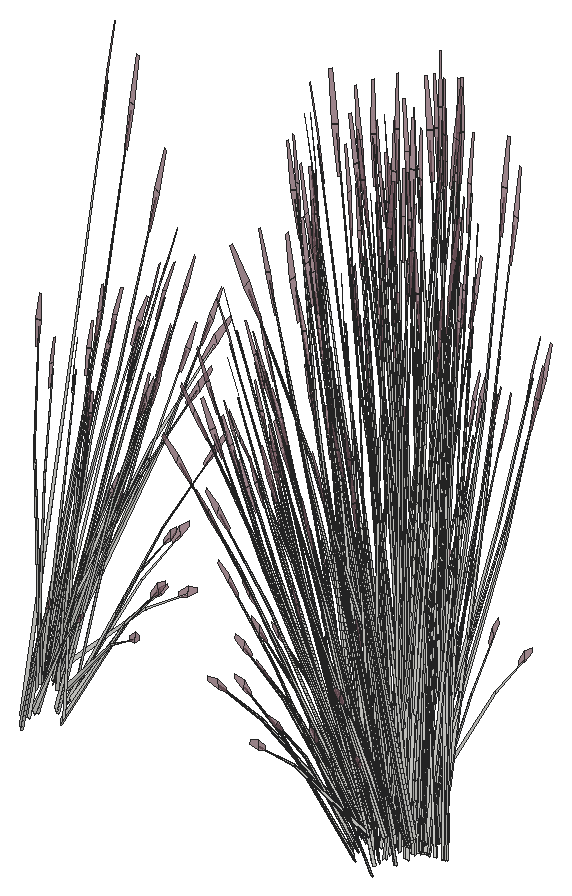
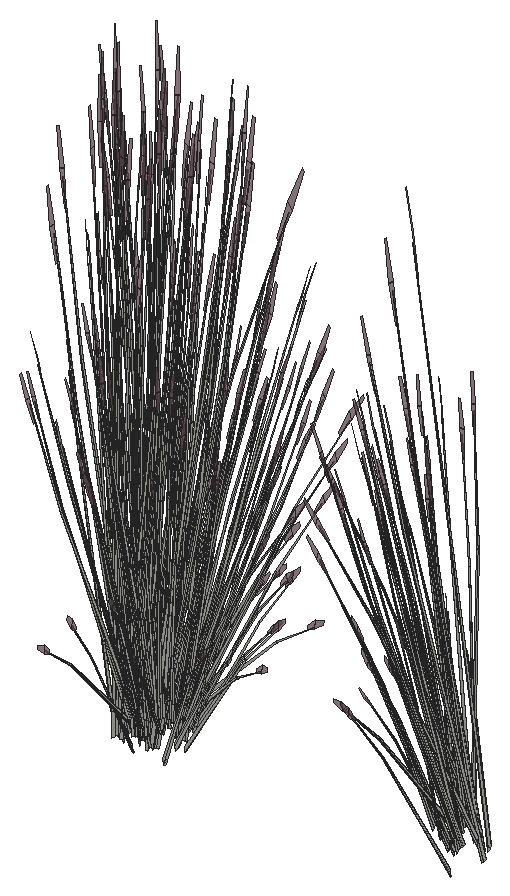
# SketchUp Ruby script. Lengths in inches.
U = 1.inch
M = Sketchup.active_model
def pt(a) = Geom::Point3d.new(a.map { |v| v * U })
def face(e, loops, mat)
  f = e.add_face(loops[0].map { |a| pt(a) })
  loops[1..].each { |l| e.add_face(l.map { |a| pt(a) }).erase! }
  f.material = f.back_material = mat if mat
  f
end
# faces: each face lists its corners as indices into pts; further lists are holes
def faces(e, pts, list, mat = nil) = list.each { |f| face(e, (f[0].is_a?(Array) ? f : [f]).map { |l| l.map { |i| pts[i] } }, mat) }
# xy, xz, yz: faces in a plane at the given z, y or x. An outline is a flat list of corners, or four numbers for a rectangle; further outlines are holes
def ring(l) = l.size == 4 ? [[l[0], l[1]], [l[2], l[1]], [l[2], l[3]], [l[0], l[3]]] : l.each_slice(2).to_a
def flat(e, list, mat, &to3) = list.each { |f| face(e, (f[0].is_a?(Array) ? f : [f]).map { |l| ring(l).map { |u, v| to3.(u, v) } }, mat) }
def xy(e, z, list, mat = nil) = flat(e, list, mat) { |x, y| [x, y, z] }
def xz(e, y, list, mat = nil) = flat(e, list, mat) { |x, z| [x, y, z] }
def yz(e, x, list, mat = nil) = flat(e, list, mat) { |y, z| [x, y, z] }
def lines(e, pts, list) = list.each { |a, b| e.add_line(pt(pts[a]), pt(pts[b])) }
# prism: a flat outline (further loops are holes) pulled along v
def prism(e, loops, v, mat = nil)
  f = face(e, loops, mat); d = Geom::Vector3d.new(v.map { |x| x * U })
  f.pushpull(f.normal.samedirection?(d) ? d.length : -d.length)
end
def box(e, o, s, mat = nil) = prism(e, [[o, [o[0] + s[0], o[1], o[2]], [o[0] + s[0], o[1] + s[1], o[2]], [o[0], o[1] + s[1], o[2]]]], [0, 0, s[2]], mat)
def at(x, y, z, deg = 0) = Geom::Transformation.translation(pt([x, y, z])) * Geom::Transformation.rotation(ORIGIN, Z_AXIS, deg.degrees)
def axes(o, x, y, z) = Geom::Transformation.new([*x, 0, *y, 0, *z, 0, *pt(o).to_a, 1])
def part(name) = M.definitions.add(name)
# library, detail: a bought-in or finely detailed component or shape, given as its bounding box
def library(name, o, s) = part(name).tap { |d| box(d.entities, o, s) }
def detail(e, o, s) = box(e.add_group.entities, o, s)
def put(e, d, t, mat = nil) = e.add_instance(d, t).tap { |i| i.material = mat if mat }
def group(e, t, mat = nil) = e.add_group.tap { |g| g.transformation = t; g.material = mat if mat }.entities
root = M.entities
M.materials.add("LightPink_Translucent").color = [144, 107, 117]
M.materials["LightPink_Translucent"].alpha = 0.75
c1 = part("blade")
p = [[2.15,0.21,22],[0,0.17,0],[0.09,0.45,0],[2.18,0.31,22],[2.29,0.31,22],[0.38,0.45,0],
  [2.48,0.24,33],[2.49,0.24,33],[2.48,0.22,33]]
faces(c1.entities,p,[[0,1,2,3],[4,5,2,3],[6,3,4,7],[8,0,3,6]])
c2 = part("seeds")
p = [[0.3,-0.1,1.38],[-0.01,-0.03,1.59],[-0.01,-0.03,0.03],[0.14,-0.07,-0.07],[0.29,-0.03,3],[0.15,0.01,3.11]]
faces(c2.entities,p,[[0,1,2,3],[1,0,4,5]],"LightPink_Translucent")
c3 = part("blade with seeds")
put(c3.entities,c1,at(0,0,0))
put(c3.entities,c2,axes([2.4,0.25,30.99],[1.5799,-0.05474,1.17369],[-0.12525,1.92788,0.29478],[-0.07173,-0.02425,1.56792]))
put(root,c3,axes([351.05,12.39,-0.97],[-0.70283,-0.33692,-0.1216],[0.40491,-0.48793,-0.67495],[0.19857,-0.16961,1.02557]))
put(root,c3,axes([349.24,15.27,-1.32],[0.74975,-0.14525,-0.51099],[0.13115,0.55007,-0.3958],[0.20138,0.15763,0.97773]))
put(root,c3,axes([349.92,10.96,-3.625],[0.47504,-0.61229,0],[0.79476,0.34146,-0.51607],[0.18101,0.07777,1.63711]))
put(root,c3,axes([350.72,10.69,-4.51],[-0.11372,-0.04814,1.76342],[-0.29211,-0.53779,-0.26939],[0.19706,-0.14594,0.30037]))
put(root,c3,axes([350.1,14.61,-0.95],[-0.43232,-0.38257,0.35414],[0.49364,-0.36215,-0.4572],[0.25081,0.0551,0.87481]))
put(root,c3,axes([350.36,11.33,-3.98],[0.7111,0.30552,-0.49651],[-0.42504,0.54784,0],[0.16196,0.06958,1.57504]))
put(root,c3,axes([350.49,14.95,-1.27],[-0.03826,0.46465,0.0643],[-0.57772,-0.01274,0.50621],[0.2213,0.04862,0.77189]))
put(root,c3,axes([350.32,15.68,-4.51],[0.05536,-0.08822,1.76342],[0.69692,-0.25981,-0.26939],[0.21129,0.13447,0.30037]))
put(root,c3,axes([350.54,14.81,-1.27],[-0.56024,0.40262,0.48003],[-0.48318,-0.42758,0.3958],[0.26285,0.07427,0.9933]))
put(root,c3,axes([350.7,11.99,-1.32],[-0.19519,-0.55794,-0.51099],[0.73919,-0.0976,-0.3958],[0.21183,-0.14986,0.97773]))
put(root,c3,axes([352,14.87,-2.07],[-0.14542,-0.51365,-0.03492],[0.68734,-0.11809,-0.15832],[0.14353,0.03256,0.52218]))
put(root,c3,axes([350.81,13.53,-0.95],[-0.63144,-0.17046,0.35414],[0.18417,-0.49731,-0.4572],[0.25423,-0.0456,0.87481]))
put(root,c3,axes([349.32,12.5,-3.94],[0.79037,0.10018,-0.62353],[-0.16679,0.61794,-0.16365],[0.23587,0.07488,1.37633]))
put(root,c3,axes([352.6875,12.86,-3.74],[-0.47106,-0.39072,-0.06488],[0.51591,-0.35801,-0.29416],[0.14618,-0.02521,0.97024]))
put(root,c3,axes([351.6,10.875,-3.23],[-0.25308,0.31105,1.1486],[-0.21753,-0.4179,0.84392],[0.20902,-0.10472,0.25299]))
put(root,c3,axes([351.3,12.26,-1.27],[0.52161,0.25698,0.0643],[-0.30368,0.36595,0.50621],[0.16723,-0.11831,0.77189]))
put(root,c3,axes([351.16,12.15,-1.27],[0.18844,0.56237,0.48003],[-0.73919,0.0976,0.3958],[0.21785,-0.13226,0.9933]))
put(root,c3,axes([349.16,13.83,-2.125],[-0.28223,-0.10528,1.71376],[0.58406,-0.44165,0.13857],[0.36402,0.19924,0.73262]))
put(root,c3,axes([352.78,12.24,-1.29],[-0.09924,-0.00464,1.77383],[-0.4121,-0.49725,-0.16761],[0.1655,-0.1635,0.31391]))
put(root,c3,axes([351.24,12.04,-1.47],[0.66138,-0.08733,-0.35414],[0.17464,0.49921,0.4572],[0.18953,-0.13408,0.87481]))
put(root,c3,axes([350.72,12.21,-1.02],[0.39688,-0.48213,-0.71045],[0.69548,0.34264,0.08574],[0.23697,-0.17468,1.00501]))
put(root,c3,axes([351.38,13.6875,-1.27],[0.27906,0.41663,0.0643],[-0.50888,0.20393,0.50621],[0.22432,-0.04024,0.77189]))
put(root,c3,axes([350.71,14.81,-1.47],[0.43232,0.38257,-0.35414],[-0.49364,0.36215,0.4572],[0.25081,0.0551,0.87481]))
put(root,c3,axes([350.22,14.85,-0.97],[0.04068,-0.62141,-0.1216],[0.77029,0.01698,-0.67495],[0.29667,0.04317,1.02557]))
put(root,c3,axes([351.07,13.7,-0.97],[-0.38229,-0.5533,-0.1216],[0.6785,-0.2719,-0.67495],[0.28593,-0.073,1.02557]))
put(root,c3,axes([351.33,13.54,-1.27],[-0.21466,0.55714,0.48003],[-0.70573,-0.19051,0.3958],[0.27753,-0.03348,0.9933]))
put(root,c3,axes([350.89,14.48,-1.28],[0.16299,-0.01033,1.74944],[0.44707,-0.47471,-0.27667],[0.28992,0.06266,0.14031]))
put(root,c3,axes([351.04,13.22,-1.32],[0.20584,-0.55581,-0.51099],[0.70573,0.19051,-0.3958],[0.28414,-0.05097,0.97773]))
put(root,c3,axes([352.8125,13.58,-3.23],[-0.46945,0.10088,1.1486],[0.22097,-0.4169,0.84392],[0.24904,0.02853,0.25299]))
put(root,c3,axes([351.29,11.77,-3.41],[-0.27143,-0.0181,1.43002],[-0.27808,-0.48551,-0.30754],[0.33346,-0.13735,0.61141]))
put(root,c3,axes([351.47,13.48,-1.47],[0.63144,0.17046,-0.35414],[-0.18417,0.49731,0.4572],[0.25423,-0.0456,0.87481]))
put(root,c3,axes([350.25,14.55,-1.02],[0.75952,0.01471,-0.71045],[-0.05101,0.61953,0.08574],[0.32177,0.06538,1.00501]))
put(root,c3,axes([351.79,13.38,-4.02],[-0.48937,0.07333,1.41583],[-0.07789,-0.58369,0.08104],[0.34275,-0.08835,0.80566]))
put(root,c3,axes([352.33,13,-4.51],[-0.03971,-0.09277,1.76342],[0.27541,-0.54264,-0.26939],[0.27782,-0.00781,0.30037]))
put(root,c3,axes([352.59,15.34,-1.29],[-0.0687,-0.05349,1.77383],[0.15029,-0.57341,-0.16761],[0.27062,-0.03664,0.31391]))
put(root,c3,axes([349.75,12.86,-2.125],[-0.31515,0.01384,1.71376],[0.20907,-0.5998,0.13857],[0.44912,0.0371,0.73262]))
put(root,c3,axes([350.91,13.43,-1.02],[0.66765,-0.26986,-0.71045],[0.37208,0.55551,0.08574],[0.32259,-0.0631,1.00501]))
put(root,c3,axes([353.15,12.83,-1.28],[0.10543,-0.09307,1.74944],[-0.13495,-0.57092,-0.27667],[0.26455,-0.10825,0.14031]))
put(root,c3,axes([351.93,14.25,-3.41],[-0.18299,-0.15028,1.43002],[0.23809,-0.49714,-0.30754],[0.37023,0.06735,0.61141]))
put(root,c3,axes([380.34,12.17,-2.125],[0.31515,-0.01384,1.71376],[-0.20907,0.5998,0.13857],[-0.44912,-0.0371,0.73262]))
put(root,c3,axes([380.47,13.23,-2.125],[0.26363,-0.12925,1.71376],[0.22195,0.59723,0.13857],[-0.41388,0.13498,0.73262]))
put(root,c3,axes([379.65,14.24,-3.41],[0.26405,0.05016,1.43002],[0.17019,0.51235,-0.30754],[-0.35868,0.0959,0.61141]))
put(root,c3,axes([381.99,12.6,-2.66],[0.21597,-0.08839,1.77064],[0.07448,0.61717,0.13857],[-0.4678,0.08189,0.63284]))
put(root,c3,axes([379.67,13.02,-1.28],[-0.12407,0.07933,1.74944],[0.01055,0.57963,-0.27667],[-0.2844,0.07538,0.14031]))
put(root,c3,axes([381.29,11.61,-1.02],[-0.75952,-0.01471,-0.71045],[0.05101,-0.61953,0.08574],[-0.32177,-0.06538,1.00501]))
put(root,c3,axes([380.67,11.76,-3.41],[0.14835,0.17012,1.43002],[-0.34183,0.46242,-0.30754],[-0.351,-0.11053,0.61141]))
put(root,c3,axes([380.07,12.6875,-1.47],[-0.63144,-0.17046,-0.35414],[0.18417,-0.49731,0.4572],[-0.25423,0.0456,0.87481]))
put(root,c3,axes([380.9375,11.21,-2.125],[0.28223,0.10528,1.71376],[-0.58406,0.44165,0.13857],[-0.36402,-0.19924,0.73262]))
put(root,c3,axes([378.29,13.6,-1.29],[0.09697,0.01639,1.77383],[0.29997,0.53988,-0.16761],[-0.1985,0.1417,0.31391]))
put(root,c3,axes([380.5,12.94,-1.32],[-0.20584,0.55581,-0.51099],[-0.70573,-0.19051,-0.3958],[-0.28414,0.05097,0.97773]))
put(root,c3,axes([381.03,11.74,-1.32],[-0.55171,0.40476,-0.51099],[-0.48318,-0.42758,-0.3958],[-0.28031,-0.06159,0.97773]))
put(root,c3,axes([380.14,12.91,-4.51],[0.01927,0.0963,1.76342],[-0.38846,0.5029,-0.26939],[-0.27592,-0.02535,0.30037]))
put(root,c3,axes([380.25,10.6,-1.29],[0.05633,0.06098,1.77383],[-0.27155,0.54815,-0.16761],[-0.27501,0.00397,0.31391]))
put(root,c3,axes([379.1,15.32,-3.23],[0.31665,-0.27694,1.1486],[0.12495,0.43841,0.84392],[-0.22883,0.0785,0.25299]))
put(root,c3,axes([380.88,10.24,-1.28],[-0.16348,-0.00431,1.74944],[-0.52047,0.43131,-0.27667],[-0.2777,-0.08813,0.14031]))
put(root,c3,axes([380.21,12.625,-1.27],[0.21466,-0.55714,0.48003],[0.70573,0.19051,0.3958],[-0.27753,0.03348,0.9933]))
put(root,c3,axes([380.46,12.46,-0.97],[0.38229,0.5533,-0.1216],[-0.6785,0.2719,-0.67495],[-0.28593,0.073,1.02557]))
put(root,c3,axes([381.32,11.32,-0.97],[-0.04068,0.62141,-0.1216],[-0.77029,-0.01698,-0.67495],[-0.29667,-0.04317,1.02557]))
put(root,c3,axes([380.83,11.36,-1.47],[-0.43232,-0.38257,-0.35414],[0.49364,-0.36215,0.4572],[-0.25081,-0.0551,0.87481]))
put(root,c3,axes([380.16,12.48,-1.27],[-0.27906,-0.41663,0.0643],[0.50888,-0.20393,0.50621],[-0.22432,0.04024,0.77189]))
put(root,c3,axes([381.4375,13.63,-2.125],[0.18977,-0.18775,1.71376],[0.47917,0.50677,0.13857],[-0.32866,0.23079,0.73262]))
put(root,c3,axes([380.3,14.12,-1.47],[-0.66138,0.08733,-0.35414],[-0.17464,-0.49921,0.4572],[-0.18953,0.13408,0.87481]))
put(root,c3,axes([379.94,15.6,-4.51],[0.10192,0.06105,1.76342],[0.17281,0.56562,-0.26939],[-0.22588,0.12062,0.30037]))
put(root,c3,axes([379.79,12.28,-3.23],[0.48508,-0.04372,1.1486],[-0.3077,0.38525,0.84392],[-0.23971,-0.05779,0.25299]))
put(root,c3,axes([380.38,14.01,-1.27],[-0.18844,-0.56237,0.48003],[0.73919,-0.0976,0.3958],[-0.21785,0.13226,0.9933]))
put(root,c3,axes([380.76,11.21,-0.91],[0.62747,-0.45094,0.53763],[0.54116,0.47889,0.4433],[-0.29439,-0.08318,1.11249]))
put(root,c3,axes([380.24,13.9,-1.27],[-0.52161,-0.25698,0.0643],[0.30368,-0.36595,0.50621],[-0.16723,0.11831,0.77189]))
put(root,c3,axes([381.3,14.09,-2.125],[0.14147,-0.21002,1.71376],[0.59349,0.43464,0.13857],[-0.26773,0.27089,0.73262]))
put(root,c3,axes([380.73,12.63,-0.95],[0.63144,0.17046,0.35414],[-0.18417,0.49731,-0.4572],[-0.25423,0.0456,0.87481]))
put(root,c3,axes([380.84,14.18,-1.32],[0.19519,0.55794,-0.51099],[-0.73919,0.0976,-0.3958],[-0.21183,0.14986,0.97773]))
put(root,c3,axes([381.05,11.21,-1.27],[0.03826,-0.46465,0.0643],[0.57772,0.01274,0.50621],[-0.2213,-0.04862,0.77189]))
put(root,c3,axes([379.6875,15.18,-1.28],[-0.01889,0.12092,1.74944],[0.53598,0.42065,-0.27667],[-0.14032,0.19892,0.14031]))
put(root,c3,axes([382.68,13.78,-3.94],[-0.79037,-0.10018,-0.62353],[0.16679,-0.61794,-0.16365],[-0.23587,-0.07488,1.37633]))
put(root,c3,axes([382.83,10.41,-0.57],[-0.50709,0.58578,-0.13619],[-0.73436,-0.33748,-0.75594],[-0.25527,-0.1655,1.14864]))
put(root,c3,axes([381.44,11.56,-0.95],[0.43232,0.38257,0.35414],[-0.49364,0.36215,-0.4572],[-0.25081,-0.0551,0.87481]))
put(root,c3,axes([382.61,10.88,-1.02],[-0.64788,-0.29534,-0.71045],[0.46044,-0.51755,0.08574],[-0.23473,-0.17635,1.00501]))
put(root,c3,axes([382.3,10.9,-1.32],[-0.74975,0.14525,-0.51099],[-0.13115,-0.55007,-0.3958],[-0.20138,-0.15763,0.97773]))
put(root,c3,axes([381.65,14.95,-3.98],[-0.7111,-0.30552,-0.49651],[0.42504,-0.54784,0],[-0.16196,-0.06958,1.57504]))
put(root,c3,axes([381.34,10.4,-4.51],[-0.0736,0.08049,1.76342],[-0.74378,0.17355,-0.26939],[-0.17968,-0.15788,0.30037]))
put(root,c3,axes([380.49,13.78,-0.97],[0.70283,0.33692,-0.1216],[-0.40491,0.48793,-0.67495],[-0.19857,0.16961,1.02557]))
put(root,c3,axes([382.08,15.32,-3.625],[-0.47504,0.61229,0],[-0.79476,-0.34146,-0.51607],[-0.18101,-0.07777,1.63711]))
put(root,c3,axes([379.33,15.24,-0.35],[0.67048,0.16311,-0.06488],[-0.20625,0.50201,-0.29416],[-0.10966,0.07622,0.97024]))
put(root,c3,axes([380.84,13.83,-0.95],[0.66138,-0.08733,0.35414],[0.17464,0.49921,-0.4572],[-0.18953,0.13408,0.87481]))
put(root,c3,axes([381.21,16.2,-3.41],[0.23977,-0.09639,1.43002],[0.59198,0.29065,-0.30754],[-0.1762,0.25149,0.61141]))
put(root,c3,axes([380.875,10.71,-3.87],[-0.21918,0.49894,-0.03893],[-0.6746,-0.15348,-0.17649],[-0.10242,-0.08161,0.58215]))
put(root,c3,axes([382.63,9.02,-1.29],[-0.01417,0.07324,1.77383],[-0.6991,0.2658,-0.16761],[-0.20573,-0.13587,0.31391]))
put(root,c3,axes([381.88,10.08,-3.41],[-0.04601,0.19989,1.43002],[-0.67263,0.16733,-0.30754],[-0.15723,-0.25836,0.61141]))
put(root,c3,axes([382.1,10.6,-2.125],[0.17368,0.19618,1.71376],[-0.80256,0.16516,0.13857],[-0.18139,-0.30799,0.73262]))
put(root,c3,axes([383.58,13.87,-3.33],[-0.76714,0.40567,-0.29095],[-0.51013,-0.57321,-0.50002],[-0.18927,-0.05821,1.59708]))
put(root,c3,axes([381.46,15.15,-1.27],[-0.54105,-0.41691,0.48003],[0.57458,-0.35956,0.3958],[-0.0998,0.1956,0.9933]))
put(root,c3,axes([382.38,10.49,-1.47],[-0.11735,-0.49217,-0.35414],[0.67083,-0.12996,0.4572],[-0.18018,-0.14104,0.87481]))
put(root,c3,axes([380.51,12.99,-3.625],[-0.95008,0,0],[0,-0.68292,-0.51607],[0,-0.15554,1.63711]))
put(root,c3,axes([381.85,14.72,-3.97],[-0.17848,-0.53243,-0.30978],[0.70886,-0.15119,0.30978],[-0.1429,-0.0614,1.38974]))
put(root,c3,axes([381.26,15.11,-1.27],[-0.62439,-0.02847,0.0643],[0.01712,-0.42991,0.50621],[-0.06534,0.16468,0.77189]))
put(root,c3,axes([381.46,15.28,-1.47],[-0.5141,0.32171,-0.35414],[-0.48666,-0.36734,0.4572],[-0.07405,0.18664,0.87481]))
put(root,c3,axes([384.09,14.3125,-3.94],[-0.51177,0.45928,-0.62353],[-0.63575,-0.41646,-0.16365],[-0.20507,0.11457,1.37633]))
put(root,c3,axes([382.78,10.89,-0.95],[0.11735,0.49217,0.35414],[-0.67083,0.12996,-0.4572],[-0.18018,-0.14104,0.87481]))
put(root,c3,axes([379.625,16.42,-1.29],[0.0862,-0.03689,1.77383],[0.71245,0.24539,-0.16761],[-0.01674,0.20431,0.31391]))
put(root,c3,axes([381.25,12.81,-3.67],[-0.70674,0.51372,0.30756],[-0.70717,-0.50832,-0.36492],[-0.02468,-0.14589,1.64885]))
put(root,c3,axes([384.16,14.22,-2.67],[0.65659,0.2464,1.51261],[-0.64324,0.53082,0.59816],[-0.28812,-0.31461,1.26806]))
put(root,c3,axes([381.65,9.76,-3.23],[0.39634,0.21267,1.1486],[-0.57721,0.12784,0.84392],[-0.1235,-0.16344,0.25299]))
put(root,c3,axes([384.44,14.05,-3.54],[-0.74193,-0.49181,-0.25192],[0.6243,-0.55226,0.5513],[-0.19979,0.05753,1.68216]))
put(root,c3,axes([383.09,13.58,-3.79],[-0.45644,-0.51287,-0.44739],[0.69137,-0.36116,0.21531],[-0.14771,-0.06346,1.43643]))
put(root,c3,axes([381.8,14.9375,-0.66],[-0.01977,0.56521,-0.7886],[-0.83252,-0.03796,0.09517],[-0.08786,0.23945,1.11556]))
put(root,c3,axes([381.79,16.53,-3.23],[-0.01966,-0.36332,1.1486],[0.49135,0.25914,0.84392],[-0.09663,0.17317,0.25299]))
put(root,c3,axes([382.48,10.31,-0.91],[0.84639,-0.15705,0.53763],[0.14689,0.61608,0.4433],[-0.19906,-0.18157,1.11249]))
put(root,c3,axes([384.07,13.95,-3.79],[-0.82508,0.03772,-0.44739],[-0.07462,-0.62614,0.21531],[-0.14771,0.06346,1.43643]))
put(root,c3,axes([382.67,10.45,-1.27],[0.34533,-0.38816,0.0643],[0.49176,0.22599,0.50621],[-0.15898,-0.12445,0.77189]))
put(root,c3,axes([382.49,15,-3.52],[0.7111,0.30552,0.49651],[-0.42504,0.54784,0],[-0.16196,-0.06958,1.57504]))
put(root,c3,axes([381.52,15.73,-2.64],[0.01669,-0.31544,1.54345],[0.75083,0.16661,0.21329],[-0.06506,0.33618,0.72882]))
put(root,c3,axes([383.16,13.875,-3.5625],[0.20138,-0.72405,-0.23429],[0.95485,0.12621,0.51271],[-0.16685,-0.09999,1.5644]))
put(root,c3,axes([383.51,14.05,-3.38],[-0.14658,0.54532,0.1448],[-0.71613,-0.09466,-0.41347],[-0.13033,-0.05599,1.26744]))
put(root,c3,axes([383.43,9.3,-1.28],[-0.11621,-0.08567,1.74944],[-0.77555,0.05431,-0.27667],[-0.12378,-0.20491,0.14031]))
put(root,c3,axes([384.93,15.57,-3.98],[-0.7111,0.30552,-0.49651],[-0.42504,-0.54784,0],[-0.16196,0.06958,1.57504]))
put(root,c3,axes([380.72,12.52,-3.98],[0,-0.61104,-0.49651],[0.85008,0,0],[0,-0.13917,1.57504]))
put(root,c3,axes([381.09,13.09,-3.52],[0,0.61104,0.49651],[-0.85008,0,0],[0,-0.13917,1.57504]))
put(root,c3,axes([384.98,15.4,-3.81],[-0.46912,-0.61443,-0.05142],[0.79476,-0.34146,0.51607],[-0.19584,0.0585,1.6363]))
put(root,c3,axes([381.97,15.125,-1],[0.54391,0.41056,-0.5672],[-0.57458,0.35956,-0.43934],[-0.08276,0.2086,1.08528]))
put(root,c3,axes([384.77,15.32,-3.97],[-0.70886,-0.15119,-0.30978],[0.17848,-0.53243,0.30978],[-0.1429,0.0614,1.38974]))
put(root,c3,axes([381.73,14.82,-0.95],[0.5141,-0.32171,0.35414],[0.48666,0.36734,-0.4572],[-0.07405,0.18664,0.87481]))
put(root,c3,axes([382.95,13.23,-3.33],[-0.85568,-0.29155,-0.29095],[0.41201,-0.61537,-0.50002],[-0.02689,-0.15109,1.59708]))
put(root,c3,axes([385.17,13.05,-3.16],[-0.02076,-0.57531,1.41272],[0.93937,0.14913,0.59816],[-0.22217,0.31481,1.3335]))
put(root,c3,axes([381.4,14.91,-0.6],[0.83505,0.03027,-0.13498],[-0.02282,0.57322,-0.74919],[-0.05801,0.22077,1.13838]))
put(root,c3,axes([381.38,15.74,-3.18],[0.69024,-0.1082,0.06507],[0.15868,0.43593,-0.86304],[-0.04376,0.22067,0.7736]))
put(root,c3,axes([384.65,13.78,-3.33],[0.08854,0.69723,-0.29095],[-0.92215,0.04216,-0.50002],[-0.16238,0.09287,1.59708]))
put(root,c3,axes([382.5625,12.61,-3.9],[-0.31203,-0.62659,-0.69835],[0.89884,-0.22566,-0.18329],[-0.03449,-0.21218,1.54149]))
put(root,c3,axes([384.61,10.62,-0.97],[-0.74352,0.28449,-0.1216],[-0.36538,-0.50492,-0.67495],[-0.0981,-0.21277,1.02557]))
put(root,c3,axes([383.97,10.64,-1.32],[-0.7469,-0.15318,-0.51099],[0.25601,-0.52518,-0.3958],[-0.06849,-0.21144,0.97773]))
put(root,c3,axes([382.59,14.54,-2.125],[-0.0186,-0.23452,1.71376],[0.80601,0.15558,0.13857],[-0.04985,0.33422,0.73262]))
put(root,c3,axes([381.09,12.54,-3.97],[0.53038,-0.38124,-0.30978],[0.53038,0.38124,0.30978],[0,-0.1228,1.38974]))
put(root,c3,axes([383.48,10.07,-3.87],[-0.52505,0.35054,-0.03893],[-0.48109,-0.38392,-0.17649],[-0.03387,-0.10878,0.58215]))
put(root,c3,axes([383.27,13.53,-3.64],[0.96033,0.12874,0.45755],[-0.19544,0.7271,0.17955],[-0.14034,-0.07021,1.58856]))
put(root,c3,axes([383.02,13.4,-3.28],[-0.36864,0.55059,0.44739],[-0.76598,-0.26498,-0.21531],[0,-0.12692,1.43643]))
put(root,c3,axes([384.24,10.74,-1.02],[-0.36264,-0.49684,-0.71045],[0.74649,-0.27689,0.08574],[-0.0848,-0.24006,1.00501]))
put(root,c3,axes([382.76,14.6875,-3.53],[0.81646,-0.16218,0.17642],[0.20161,0.60355,0.35086],[-0.07282,-0.08794,1.60407]))
put(root,c3,axes([383.81,14.78,-3.8],[-0.76598,-0.27433,0],[0.36864,-0.57001,0],[0,0,1.62707]))
put(root,c3,axes([384.38,10.82,-0.95],[-0.22906,0.4699,0.35414],[-0.66828,-0.13705,-0.4572],[-0.06128,-0.18919,0.87481]))
put(root,c3,axes([385.58,15.47,-3.625],[0.47504,0.61229,0],[-0.79476,0.34146,-0.51607],[-0.18101,0.07777,1.63711]))
put(root,c3,axes([383.16,15.73,-0.9375],[-0.74868,-0.15974,0.53283],[0.25601,-0.52518,0.43934],[0.04499,0.20653,1.10256]))
put(root,c3,axes([382.96,15.77,-1.27],[-0.55987,0.20767,0.0643],[-0.27403,-0.37869,0.50621],[0.05407,0.16693,0.77189]))
put(root,c3,axes([385.1875,14.72,-3.53],[0.21949,-0.60727,0.17642],[0.8032,0.17185,0.35086],[-0.13875,0.00296,1.60407]))
put(root,c3,axes([384.81,13.92,-3.38],[0.56134,0.36712,0.1448],[-0.46823,0.41419,-0.41347],[-0.13033,0.05599,1.26744]))
put(root,c3,axes([384.61,13.46,-3.7],[-0.70674,-0.52593,-0.06131],[0.70717,-0.52625,0],[-0.02468,-0.01837,1.75571]))
put(root,c3,axes([384.8,13.65,-3.28],[0.82508,-0.03772,0.44739],[0.07462,0.62614,-0.21531],[-0.14771,0.06346,1.43643]))
put(root,c3,axes([385,15.09,-3.67],[0.95122,0.19861,0.30756],[-0.23797,0.7099,-0.36492],[-0.15744,0.08885,1.64885]))
put(root,c3,axes([383.61,9.64,-4.51],[-0.12744,0.02202,1.76342],[-0.70477,-0.24781,-0.26939],[0.01183,-0.2067,0.30037]))
put(root,c3,axes([385.41,15.05,-3.52],[0.7111,-0.30552,0.49651],[0.42504,0.54784,0],[-0.16196,0.06958,1.57504]))
put(root,c3,axes([384.31,10.32,-1.47],[0.22906,-0.4699,-0.35414],[0.66828,0.13705,0.4572],[-0.06128,-0.18919,0.87481]))
put(root,c3,axes([383.1875,12.86,-3.64],[0.33034,0.68327,0.45755],[-0.94388,0.2376,0.17955],[0.01154,-0.12555,1.58856]))
put(root,c3,axes([383.04,12.77,-3.79],[0.36864,-0.55059,-0.44739],[0.76598,0.26498,0.21531],[0,-0.12692,1.43643]))
put(root,c3,axes([383.98,14.55,-3.8],[-0.24791,-0.5268,0],[0.70791,-0.18448,0],[0,0,1.54371]))
put(root,c3,axes([383.08,15.66,-4.51],[0.12297,-0.03325,1.76342],[0.73967,0.18301,-0.26939],[0.02163,0.20626,0.30037]))
put(root,c3,axes([383.24,15.84,-1.47],[-0.22906,0.4699,-0.35414],[-0.66828,-0.13705,0.4572],[0.06128,0.18919,0.87481]))
put(root,c3,axes([384.98,13.51,-3.79],[-0.36864,0.55059,-0.44739],[-0.76598,-0.26498,0.21531],[0,0.12692,1.43643]))
put(root,c3,axes([384.59,10.39,-1.27],[0.55987,-0.20767,0.0643],[0.27403,0.37869,0.50621],[-0.05407,-0.16693,0.77189]))
put(root,c3,axes([382.77,16.68,-1.28],[0.09631,0.0984,1.74944],[0.77725,0.03866,-0.27667],[0.07816,0.217,0.14031]))
put(root,c3,axes([386.4375,13.17,-3.53],[-0.59697,-0.44509,0.17642],[0.60159,-0.4317,0.35086],[-0.06593,0.0909,1.60407]))
put(root,c3,axes([384.38,12.92,-3.79],[0,-0.70701,0],[0.95008,0,0],[0,0,1.79456]))
put(root,c3,axes([384.39,10.43,-1.27],[0.74868,0.15974,0.48003],[-0.25601,0.52518,0.3958],[-0.04499,-0.20653,0.9933]))
put(root,c3,axes([383.49,13.04,-3.57],[0.8561,0.29616,0.24065],[-0.41201,0.61537,0.50002],[0,-0.14185,1.60543]))
put(root,c3,axes([384.85,13.2,-3.71],[0,0.70667,-0.05637],[-0.95008,0,0],[0,0.02221,1.79368]))
put(root,c3,axes([383.22,12.63,-3.28],[-0.82508,0.03772,0.44739],[-0.07462,-0.62614,-0.21531],[0.14771,-0.06346,1.43643]))
put(root,c3,axes([383.17,15.35,-0.95],[0.22906,-0.4699,0.35414],[0.66828,0.13705,-0.4572],[0.06128,0.18919,0.87481]))
put(root,c3,axes([382.83,11.56,-3.53],[-0.21949,0.60727,0.17642],[-0.8032,-0.17185,0.35086],[0.13875,-0.00296,1.60407]))
put(root,c3,axes([384.4,14.57,-3.71],[0.33034,0.70197,-0.06012],[-0.94388,0.24598,0],[0.01154,0.02451,1.72173]))
put(root,c3,axes([382.44,10.81,-3.625],[-0.47504,-0.61229,0],[0.79476,-0.34146,-0.51607],[0.18101,-0.07777,1.63711]))
put(root,c3,axes([383.3125,15.42,-1.02],[0.36264,0.49684,-0.71045],[-0.74649,0.27689,0.08574],[0.0848,0.24006,1.00501]))
put(root,c3,axes([387.13,13.64,-3.8],[-0.94962,-0.00489,-0.04976],[0,-0.68292,0.49943],[-0.02984,0.15546,1.58352]))
put(root,c3,axes([385.26,11.59,-3.53],[-0.81646,0.16218,0.17642],[-0.20161,-0.60355,0.35086],[0.07282,0.08794,1.60407]))
put(root,c3,axes([384.43,9.33,-3.23],[0.09747,0.35631,1.1486],[-0.54071,-0.19735,0.84392],[0.05818,-0.18244,0.25299]))
put(root,c3,axes([384.07,17.03,-0.35],[0.52505,-0.35054,-0.06488],[0.48109,0.38392,-0.29416],[0.03387,0.10878,0.97024]))
put(root,c3,axes([383.93,12.47,-3.64],[-0.62999,0.55453,0.45755],[-0.74845,-0.4895,0.17955],[0.15188,-0.05534,1.58856]))
put(root,c3,axes([385,13.34,-3.79],[0.53038,0.39469,0],[-0.53038,0.39469,0],[0,0,1.69266]))
put(root,c3,axes([385,12.88,-3.28],[0.36864,-0.55059,0.44739],[0.76598,0.26498,-0.21531],[0,0.12692,1.43643]))
put(root,c3,axes([384.68,14.8,-3.8],[0.76598,0.27433,0],[-0.36864,0.57001,0],[0,0,1.74954]))
put(root,c3,axes([383.58,15.52,-1.32],[0.7469,0.15318,-0.51099],[-0.25601,0.52518,-0.3958],[0.06849,0.21144,0.97773]))
put(root,c3,axes([382.95,15.55,-0.97],[0.74352,-0.28449,-0.1216],[0.36538,0.50492,-0.67495],[0.0981,0.21277,1.02557]))
put(root,c3,axes([384.75,12.75,-3.62],[-0.96033,-0.12874,0.49198],[0.19544,-0.7271,0.19306],[0.14034,0.07021,1.70813]))
put(root,c3,axes([386.74,9.91,-1.29],[-0.07716,0.04667,1.77383],[-0.75601,-0.15746,-0.16761],[-0.02737,-0.20368,0.31391]))
put(root,c3,axes([386.15,11.26,-0.97],[-0.83505,-0.03027,-0.1216],[0.02282,-0.57322,-0.67495],[0.05801,-0.22077,1.02557]))
put(root,c3,axes([386.93,13.74,-3.97],[-0.53038,0.38124,-0.30978],[-0.53038,-0.38124,0.30978],[0,0.1228,1.38974]))
put(root,c3,axes([385.42,13.67,-3.91],[0.2786,0.55945,-0.69212],[-0.80253,0.20149,-0.18165],[0.03079,0.18945,1.52773]))
put(root,c3,axes([385.02,13.07,-3.79],[0.85008,0,0],[0,0.63259,0],[0,0,1.78407]))
put(root,c3,axes([385.82,11.35,-0.95],[-0.5141,0.32171,0.35414],[-0.48666,-0.36734,-0.4572],[0.07405,-0.18664,0.87481]))
put(root,c3,axes([384.2,12.375,-3.28],[-0.45644,-0.51287,0.44739],[0.69137,-0.36116,-0.21531],[0.14771,0.06346,1.43643]))
put(root,c3,axes([383.375,12.5,-3.33],[-0.08854,-0.69723,-0.29095],[0.92215,-0.04216,-0.50002],[0.16238,-0.09287,1.59708]))
put(root,c3,axes([385.32,13.01,-3.38],[0.70791,-0.1782,0.1448],[0.24791,0.50885,-0.41347],[0,0.11199,1.26744]))
put(root,c3,axes([385.58,11.04,-1.32],[-0.54391,-0.41056,-0.51099],[0.57458,-0.35956,-0.3958],[0.08276,-0.2086,0.97773]))
put(root,c3,axes([385.07,13.05,-3.33],[0.85568,0.29155,-0.29095],[-0.41201,0.61537,-0.50002],[0.02689,0.15109,1.59708]))
put(root,c3,axes([383.25,10.95,-3.97],[0.70886,0.15119,-0.30978],[-0.17848,0.53243,0.30978],[0.1429,-0.0614,1.38974]))
put(root,c3,axes([385.22,10.3125,-3.41],[-0.21597,0.12368,1.43002],[-0.64681,-0.21647,-0.30754],[0.1199,-0.26922,0.61141]))
put(root,c3,axes([386.93,13.19,-3.52],[0,-0.61104,0.49651],[0.85008,0,0],[0,0.13917,1.57504]))
